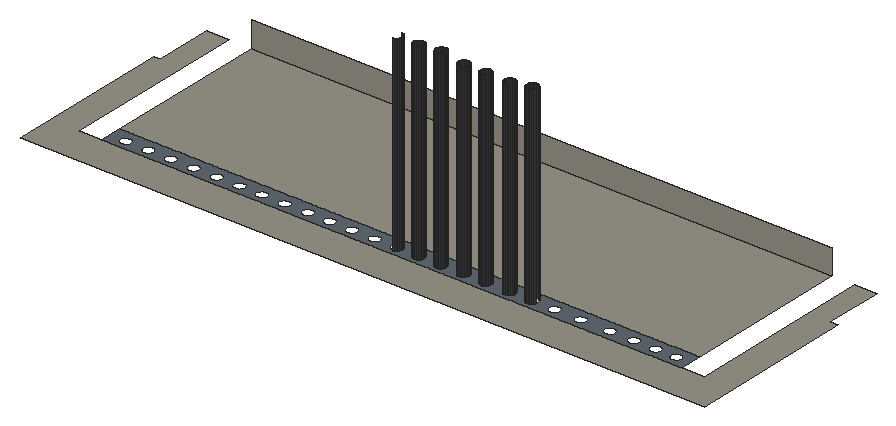
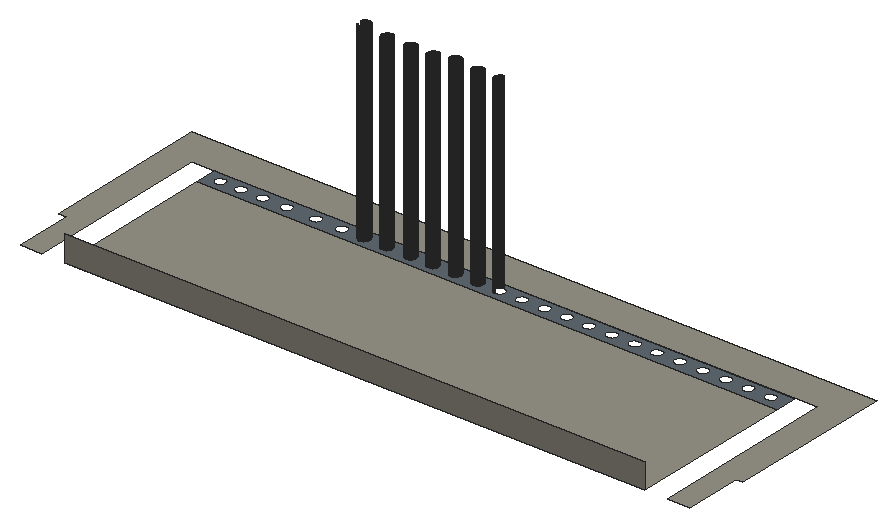
# SketchUp Ruby script. Lengths in inches.
U = 1.inch
M = Sketchup.active_model
def pt(a) = Geom::Point3d.new(a.map { |v| v * U })
def face(e, loops, mat)
  f = e.add_face(loops[0].map { |a| pt(a) })
  loops[1..].each { |l| e.add_face(l.map { |a| pt(a) }).erase! }
  f.material = f.back_material = mat if mat
  f
end
# faces: each face lists its corners as indices into pts; further lists are holes
def faces(e, pts, list, mat = nil) = list.each { |f| face(e, (f[0].is_a?(Array) ? f : [f]).map { |l| l.map { |i| pts[i] } }, mat) }
# xy, xz, yz: faces in a plane at the given z, y or x. An outline is a flat list of corners, or four numbers for a rectangle; further outlines are holes
def ring(l) = l.size == 4 ? [[l[0], l[1]], [l[2], l[1]], [l[2], l[3]], [l[0], l[3]]] : l.each_slice(2).to_a
def flat(e, list, mat, &to3) = list.each { |f| face(e, (f[0].is_a?(Array) ? f : [f]).map { |l| ring(l).map { |u, v| to3.(u, v) } }, mat) }
def xy(e, z, list, mat = nil) = flat(e, list, mat) { |x, y| [x, y, z] }
def xz(e, y, list, mat = nil) = flat(e, list, mat) { |x, z| [x, y, z] }
def yz(e, x, list, mat = nil) = flat(e, list, mat) { |y, z| [x, y, z] }
def lines(e, pts, list) = list.each { |a, b| e.add_line(pt(pts[a]), pt(pts[b])) }
# prism: a flat outline (further loops are holes) pulled along v
def prism(e, loops, v, mat = nil)
  f = face(e, loops, mat); d = Geom::Vector3d.new(v.map { |x| x * U })
  f.pushpull(f.normal.samedirection?(d) ? d.length : -d.length)
end
def box(e, o, s, mat = nil) = prism(e, [[o, [o[0] + s[0], o[1], o[2]], [o[0] + s[0], o[1] + s[1], o[2]], [o[0], o[1] + s[1], o[2]]]], [0, 0, s[2]], mat)
def at(x, y, z, deg = 0) = Geom::Transformation.translation(pt([x, y, z])) * Geom::Transformation.rotation(ORIGIN, Z_AXIS, deg.degrees)
def axes(o, x, y, z) = Geom::Transformation.new([*x, 0, *y, 0, *z, 0, *pt(o).to_a, 1])
def part(name) = M.definitions.add(name)
# library, detail: a bought-in or finely detailed component or shape, given as its bounding box
def library(name, o, s) = part(name).tap { |d| box(d.entities, o, s) }
def detail(e, o, s) = box(e.add_group.entities, o, s)
def put(e, d, t, mat = nil) = e.add_instance(d, t).tap { |i| i.material = mat if mat }
def group(e, t, mat = nil) = e.add_group.tap { |g| g.transformation = t; g.material = mat if mat }.entities
root = M.entities
M.materials.add("[Color M07]").color = [58, 58, 58]
M.materials.add("[Formica Graystone]").color = [149, 146, 135]
M.materials.add("[Formica Speckled Grey]").color = [94, 105, 111]
xy(root,334.79,[[262.29,121.51,262.12,121.56,261.96,121.65,261.84,121.78,261.75,121.93,261.71,122.11,261.71,122.28,261.76,122.46,261.85,122.61,261.98,122.74,262.13,122.83,262.31,122.87,262.48,122.87,262.66,122.82,262.8125,122.73,262.9375,122.6,263.03,122.45,263.07,122.27,263.07,122.09,263.02,121.92,262.93,121.76,262.8,121.64,262.65,121.55,262.47,121.51],[265.04,121.51,264.87,121.56,264.71,121.65,264.59,121.78,264.5,121.93,264.46,122.11,264.46,122.28,264.51,122.46,264.6,122.61,264.73,122.74,264.88,122.83,265.06,122.87,265.23,122.87,265.41,122.82,265.5625,122.73,265.6875,122.6,265.78,122.45,265.82,122.27,265.82,122.09,265.77,121.92,265.68,121.76,265.55,121.64,265.4,121.55,265.22,121.51],[267.79,121.51,267.62,121.56,267.46,121.65,267.34,121.78,267.25,121.93,267.21,122.11,267.21,122.28,267.26,122.46,267.35,122.61,267.48,122.74,267.63,122.83,267.81,122.87,267.98,122.87,268.16,122.82,268.3125,122.73,268.4375,122.6,268.53,122.45,268.57,122.27,268.57,122.09,268.52,121.92,268.43,121.76,268.3,121.64,268.15,121.55,267.97,121.51],[270.54,121.51,270.37,121.56,270.21,121.65,270.09,121.78,270,121.93,269.96,122.11,269.96,122.28,270.01,122.46,270.1,122.61,270.23,122.74,270.38,122.83,270.56,122.87,270.73,122.87,270.91,122.82,271.0625,122.73,271.1875,122.6,271.28,122.45,271.32,122.27,271.32,122.09,271.27,121.92,271.18,121.76,271.05,121.64,270.9,121.55,270.72,121.51],[273.48,121.51,273.31,121.56,273.15,121.65,273.03,121.78,272.9375,121.93,272.89,122.11,272.9,122.28,272.94,122.46,273.03,122.61,273.16,122.74,273.32,122.83,273.49,122.87,273.67,122.87,273.85,122.82,274,122.73,274.125,122.6,274.21,122.45,274.26,122.27,274.26,122.09,274.21,121.92,274.12,121.76,273.99,121.64,273.83,121.55,273.66,121.51],
  [276.29,121.51,276.12,121.56,275.96,121.65,275.84,121.78,275.75,121.93,275.71,122.11,275.71,122.28,275.76,122.46,275.85,122.61,275.98,122.74,276.13,122.83,276.31,122.87,276.48,122.87,276.66,122.82,276.8125,122.73,276.9375,122.6,277.03,122.45,277.07,122.27,277.07,122.09,277.02,121.92,276.93,121.76,276.8,121.64,276.65,121.55,276.47,121.51]])
xy(root,334.79,[[217.8,116.35,302.43,116.35,302.43,136.91,301.43,136.91,301.43,144.04,298.73,144.04,298.73,120.91,221.4,120.91,221.4,144.04,218.68,144.04,218.68,136.91,217.8,136.91],[224.22,123.73,295.92,144.04]],"[Formica Graystone]")
xy(root,334.79,[[[224.22,120.91,295.92,123.73],[228.85,121.51,228.68,121.56,228.53,121.65,228.4,121.78,228.3125,121.93,228.27,122.11,228.27,122.28,228.32,122.46,228.41,122.61,228.54,122.74,228.69,122.83,228.87,122.87,229.05,122.87,229.22,122.82,229.375,122.73,229.5,122.6,229.59,122.45,229.63,122.27,229.63,122.09,229.58,121.92,229.49,121.76,229.36,121.64,229.21,121.55,229.03,121.51],[231.67,121.51,231.49,121.56,231.34,121.65,231.21,121.78,231.125,121.93,231.08,122.11,231.08,122.28,231.13,122.46,231.22,122.61,231.35,122.74,231.51,122.83,231.68,122.87,231.86,122.87,232.03,122.82,232.1875,122.73,232.3125,122.6,232.4,122.45,232.45,122.27,232.44,122.09,232.4,121.92,232.3,121.76,232.18,121.64,232.02,121.55,231.85,121.51],[234.48,121.51,234.31,121.56,234.15,121.65,234.03,121.78,233.9375,121.93,233.89,122.11,233.9,122.28,233.94,122.46,234.03,122.61,234.16,122.74,234.32,122.83,234.49,122.87,234.67,122.87,234.85,122.82,235,122.73,235.125,122.6,235.21,122.45,235.26,122.27,235.26,122.09,235.21,121.92,235.12,121.76,234.99,121.64,234.83,121.55,234.66,121.51],[237.29,121.51,237.12,121.56,236.96,121.65,236.84,121.78,236.75,121.93,236.71,122.11,236.71,122.28,236.76,122.46,236.85,122.61,236.98,122.74,237.13,122.83,237.31,122.87,237.48,122.87,237.66,122.82,237.8125,122.73,237.9375,122.6,238.03,122.45,238.07,122.27,238.07,122.09,238.02,121.92,237.93,121.76,237.8,121.64,237.65,121.55,237.47,121.51],[240.1,121.51,239.93,121.56,239.78,121.65,239.65,121.78,239.5625,121.93,239.52,122.11,239.52,122.28,239.57,122.46,239.66,122.61,239.79,122.74,239.94,122.83,240.12,122.87,240.3,122.87,240.47,122.82,240.625,122.73,240.75,122.6,240.84,122.45,240.88,122.27,240.88,122.09,240.83,121.92,240.74,121.76,240.61,121.64,240.46,121.55,240.28,121.51],[242.92,121.51,242.74,121.56,242.59,121.65,242.46,121.78,242.375,121.93,242.33,122.11,242.33,122.28,242.38,122.46,242.47,122.61,242.6,122.74,242.76,122.83,242.93,122.87,243.11,122.87,243.28,122.82,243.4375,122.73,243.5625,122.6,243.65,122.45,243.7,122.27,243.69,122.09,243.65,121.92,243.55,121.76,243.43,121.64,243.27,121.55,243.1,121.51],[245.73,121.51,245.56,121.56,245.4,121.65,245.28,121.78,245.1875,121.93,245.14,122.11,245.15,122.28,245.19,122.46,245.28,122.61,245.41,122.74,245.57,122.83,245.74,122.87,245.92,122.87,246.1,122.82,246.25,122.73,246.375,122.6,246.46,122.45,246.51,122.27,246.51,122.09,246.46,121.92,246.37,121.76,246.24,121.64,246.08,121.55,245.91,121.51],[248.54,121.51,248.37,121.56,248.21,121.65,248.09,121.78,248,121.93,247.96,122.11,247.96,122.28,248.01,122.46,248.1,122.61,248.23,122.74,248.38,122.83,248.56,122.87,248.73,122.87,248.91,122.82,249.0625,122.73,249.1875,122.6,249.28,122.45,249.32,122.27,249.32,122.09,249.27,121.92,249.18,121.76,249.05,121.64,248.9,121.55,248.72,121.51],[251.29,121.51,251.12,121.56,250.96,121.65,250.84,121.78,250.75,121.93,250.71,122.11,250.71,122.28,250.76,122.46,250.85,122.61,250.98,122.74,251.13,122.83,251.31,122.87,251.48,122.87,251.66,122.82,251.8125,122.73,251.9375,122.6,252.03,122.45,252.07,122.27,252.07,122.09,252.02,121.92,251.93,121.76,251.8,121.64,251.65,121.55,251.47,121.51],[254.04,121.51,253.87,121.56,253.71,121.65,253.59,121.78,253.5,121.93,253.46,122.11,253.46,122.28,253.51,122.46,253.6,122.61,253.73,122.74,253.88,122.83,254.06,122.87,254.23,122.87,254.41,122.82,254.5625,122.73,254.6875,122.6,254.78,122.45,254.82,122.27,254.82,122.09,254.77,121.92,254.68,121.76,254.55,121.64,254.4,121.55,254.22,121.51],[256.79,121.51,256.62,121.56,256.46,121.65,256.34,121.78,256.25,121.93,256.21,122.11,256.21,122.28,256.26,122.46,256.35,122.61,256.48,122.74,256.63,122.83,256.81,122.87,256.98,122.87,257.16,122.82,257.3125,122.73,257.4375,122.6,257.53,122.45,257.57,122.27,257.57,122.09,257.52,121.92,257.43,121.76,257.3,121.64,257.15,121.55,256.97,121.51],[259.54,121.51,259.37,121.56,259.21,121.65,259.09,121.78,259,121.93,258.96,122.11,258.96,122.28,259.01,122.46,259.1,122.61,259.23,122.74,259.38,122.83,259.56,122.87,259.73,122.87,259.91,122.82,260.0625,122.73,260.1875,122.6,260.28,122.45,260.32,122.27,260.32,122.09,260.27,121.92,260.18,121.76,260.05,121.64,259.9,121.55,259.72,121.51],[262.29,121.51,262.12,121.56,261.96,121.65,261.84,121.78,261.75,121.93,261.71,122.11,261.71,122.28,261.76,122.46,261.85,122.61,261.98,122.74,262.13,122.83,262.31,122.87,262.48,122.87,262.66,122.82,262.8125,122.73,262.9375,122.6,263.03,122.45,263.07,122.27,263.07,122.09,263.02,121.92,262.93,121.76,262.8,121.64,262.65,121.55,262.47,121.51],[265.04,121.51,264.87,121.56,264.71,121.65,264.59,121.78,264.5,121.93,264.46,122.11,264.46,122.28,264.51,122.46,264.6,122.61,264.73,122.74,264.88,122.83,265.06,122.87,265.23,122.87,265.41,122.82,265.5625,122.73,265.6875,122.6,265.78,122.45,265.82,122.27,265.82,122.09,265.77,121.92,265.68,121.76,265.55,121.64,265.4,121.55,265.22,121.51],[267.79,121.51,267.62,121.56,267.46,121.65,267.34,121.78,267.25,121.93,267.21,122.11,267.21,122.28,267.26,122.46,267.35,122.61,267.48,122.74,267.63,122.83,267.81,122.87,267.98,122.87,268.16,122.82,268.3125,122.73,268.4375,122.6,268.53,122.45,268.57,122.27,268.57,122.09,268.52,121.92,268.43,121.76,268.3,121.64,268.15,121.55,267.97,121.51],[270.54,121.51,270.37,121.56,270.21,121.65,270.09,121.78,270,121.93,269.96,122.11,269.96,122.28,270.01,122.46,270.1,122.61,270.23,122.74,270.38,122.83,270.56,122.87,270.73,122.87,270.91,122.82,271.0625,122.73,271.1875,122.6,271.28,122.45,271.32,122.27,271.32,122.09,271.27,121.92,271.18,121.76,271.05,121.64,270.9,121.55,270.72,121.51],[294.1,121.51,293.93,121.56,293.78,121.65,293.65,121.78,293.5625,121.93,293.52,122.11,293.52,122.28,293.57,122.46,293.66,122.61,293.79,122.74,293.94,122.83,294.12,122.87,294.3,122.87,294.47,122.82,294.625,122.73,294.75,122.6,294.84,122.45,294.88,122.27,294.88,122.09,294.83,121.92,294.74,121.76,294.61,121.64,294.46,121.55,294.28,121.51],[273.48,121.51,273.31,121.56,273.15,121.65,273.03,121.78,272.9375,121.93,272.89,122.11,272.9,122.28,272.94,122.46,273.03,122.61,273.16,122.74,273.32,122.83,273.49,122.87,273.67,122.87,273.85,122.82,274,122.73,274.125,122.6,274.21,122.45,274.26,122.27,274.26,122.09,274.21,121.92,274.12,121.76,273.99,121.64,273.83,121.55,273.66,121.51],[291.54,121.51,291.37,121.56,291.21,121.65,291.09,121.78,291,121.93,290.96,122.11,290.96,122.28,291.01,122.46,291.1,122.61,291.23,122.74,291.38,122.83,291.56,122.87,291.73,122.87,291.91,122.82,292.0625,122.73,292.1875,122.6,292.28,122.45,292.32,122.27,292.32,122.09,292.27,121.92,292.18,121.76,292.05,121.64,291.9,121.55,291.72,121.51],[276.29,121.51,276.12,121.56,275.96,121.65,275.84,121.78,275.75,121.93,275.71,122.11,275.71,122.28,275.76,122.46,275.85,122.61,275.98,122.74,276.13,122.83,276.31,122.87,276.48,122.87,276.66,122.82,276.8125,122.73,276.9375,122.6,277.03,122.45,277.07,122.27,277.07,122.09,277.02,121.92,276.93,121.76,276.8,121.64,276.65,121.55,276.47,121.51],[288.85,121.51,288.68,121.56,288.53,121.65,288.4,121.78,288.3125,121.93,288.27,122.11,288.27,122.28,288.32,122.46,288.41,122.61,288.54,122.74,288.69,122.83,288.87,122.87,289.05,122.87,289.22,122.82,289.375,122.73,289.5,122.6,289.59,122.45,289.63,122.27,289.63,122.09,289.58,121.92,289.49,121.76,289.36,121.64,289.21,121.55,289.03,121.51],[279.04,121.51,278.87,121.56,278.71,121.65,278.59,121.78,278.5,121.93,278.46,122.11,278.46,122.28,278.51,122.46,278.6,122.61,278.73,122.74,278.88,122.83,279.06,122.87,279.23,122.87,279.41,122.82,279.5625,122.73,279.6875,122.6,279.78,122.45,279.82,122.27,279.82,122.09,279.77,121.92,279.68,121.76,279.55,121.64,279.4,121.55,279.22,121.51],[285.92,121.51,285.74,121.56,285.59,121.65,285.46,121.78,285.375,121.93,285.33,122.11,285.33,122.28,285.38,122.46,285.47,122.61,285.6,122.74,285.76,122.83,285.93,122.87,286.11,122.87,286.28,122.82,286.4375,122.73,286.5625,122.6,286.65,122.45,286.7,122.27,286.69,122.09,286.65,121.92,286.55,121.76,286.43,121.64,286.27,121.55,286.1,121.51],[282.29,121.51,282.12,121.56,281.96,121.65,281.84,121.78,281.75,121.93,281.71,122.11,281.71,122.28,281.76,122.46,281.85,122.61,281.98,122.74,282.13,122.83,282.31,122.87,282.48,122.87,282.66,122.82,282.8125,122.73,282.9375,122.6,283.03,122.45,283.07,122.27,283.07,122.09,283.02,121.92,282.93,121.76,282.8,121.64,282.65,121.55,282.47,121.51],[226.04,121.51,225.87,121.56,225.71,121.65,225.59,121.78,225.5,121.93,225.46,122.11,225.46,122.28,225.51,122.46,225.6,122.61,225.73,122.74,225.88,122.83,226.06,122.87,226.23,122.87,226.41,122.82,226.5625,122.73,226.6875,122.6,226.78,122.45,226.82,122.27,226.82,122.09,226.77,121.92,226.68,121.76,226.55,121.64,226.4,121.55,226.22,121.51]]],"[Formica Speckled Grey]")
xz(root,121.51,[[262.29,334.79,262.47,358.31],[265.04,334.79,265.22,358.53],[267.79,334.79,267.97,358.07],[270.54,334.79,270.72,358.07],[273.48,334.79,273.66,358.07],
  [276.29,334.79,276.47,358.53]],"[Color M07]")
xz(root,122.87,[[262.31,334.79,262.48,358.31],[265.06,334.79,265.23,358.53],[267.81,334.79,267.98,358.07],[270.56,334.79,270.73,358.07],[273.49,334.79,273.67,358.07],
  [276.31,334.79,276.48,358.53]],"[Color M07]")
xz(root,144.04,[[224.22,334.79,295.92,337.93]],"[Formica Graystone]")
yz(root,260.32,[[122.09,334.79,122.27,358.31]],"[Color M07]")
yz(root,261.71,[[122.11,334.79,122.28,358.31]],"[Color M07]")
yz(root,263.07,[[122.09,334.79,122.27,358.31]],"[Color M07]")
yz(root,264.46,[[122.11,334.79,122.28,358.53]],"[Color M07]")
yz(root,265.82,[[122.09,334.79,122.27,358.53]],"[Color M07]")
yz(root,267.21,[[122.11,334.79,122.28,358.07]],"[Color M07]")
yz(root,268.57,[[122.09,334.79,122.27,358.07]],"[Color M07]")
yz(root,269.96,[[122.11,334.79,122.28,358.07]],"[Color M07]")
yz(root,271.32,[[122.09,334.79,122.27,358.07]],"[Color M07]")
yz(root,274.26,[[122.09,334.79,122.27,358.07]],"[Color M07]")
yz(root,275.71,[[122.11,334.79,122.28,358.53]],"[Color M07]")
p = [[259.72,121.51,334.79],[259.9,121.55,334.79],[259.9,121.55,358.31],[259.72,121.51,358.31],[262.12,121.56,334.79],[262.29,121.51,334.79],
  [262.29,121.51,358.31],[262.12,121.56,358.31],[262.12,121.56,357.4],[262.47,121.51,334.79],[262.65,121.55,334.79],[262.65,121.55,358.31],
  [262.47,121.51,358.31],[264.87,121.56,334.79],[265.04,121.51,334.79],[265.04,121.51,358.53],[264.87,121.56,358.53],[264.87,121.56,357.4],
  [265.22,121.51,334.79],[265.4,121.55,334.79],[265.4,121.55,358.53],[265.22,121.51,358.53],[267.62,121.56,334.79],[267.79,121.51,334.79],
  [267.79,121.51,358.07],[267.62,121.56,358.07],[267.62,121.56,357.4],[267.97,121.51,334.79],[268.15,121.55,334.79],[268.15,121.55,358.07],
  [267.97,121.51,358.07],[270.37,121.56,334.79],[270.54,121.51,334.79],[270.54,121.51,358.07],[270.37,121.56,358.07],[270.37,121.56,357.4],
  [270.72,121.51,334.79],[270.9,121.55,334.79],[270.9,121.55,358.07],[270.72,121.51,358.07],[273.31,121.56,334.79],[273.48,121.51,334.79],
  [273.48,121.51,358.07],[273.31,121.56,358.07],[273.31,121.56,357.4],[273.66,121.51,334.79],[273.83,121.55,334.79],[273.83,121.55,358.07],
  [273.66,121.51,358.07],[276.12,121.56,334.79],[276.29,121.51,334.79],[276.29,121.51,358.53],[276.12,121.56,358.53],[276.12,121.56,357.4],
  [276.47,121.51,334.79],[276.65,121.55,334.79],[276.65,121.55,358.53],[276.47,121.51,358.53],[260.05,121.64,334.79],[260.05,121.64,358.31],
  [260.18,121.76,334.79],[260.18,121.76,358.31],[261.84,121.78,334.79],[261.96,121.65,334.79],[261.96,121.65,358.31],[261.84,121.78,358.31],
  [262.8,121.64,334.79],[262.8,121.64,358.31],[262.93,121.76,334.79],[262.93,121.76,358.31],[264.59,121.78,334.79],[264.71,121.65,334.79],
  [264.71,121.65,358.53],[264.59,121.78,358.53],[265.55,121.64,334.79],[265.55,121.64,358.53],[265.68,121.76,334.79],[265.68,121.76,358.53],
  [267.34,121.78,334.79],[267.46,121.65,334.79],[267.46,121.65,358.07],[267.34,121.78,358.07],[268.3,121.64,334.79],[268.3,121.64,358.07],
  [268.43,121.76,334.79],[268.43,121.76,358.07],[270.09,121.78,334.79],[270.21,121.65,334.79],[270.21,121.65,358.07],[270.09,121.78,358.07],
  [271.05,121.64,334.79],[271.05,121.64,358.07],[271.18,121.76,334.79],[271.18,121.76,358.07],[273.03,121.78,334.79],[273.15,121.65,334.79],
  [273.15,121.65,358.07],[273.03,121.78,358.07],[273.99,121.64,334.79],[273.99,121.64,358.07],[274.12,121.76,334.79],[274.12,121.76,358.07],
  [275.84,121.78,334.79],[275.96,121.65,334.79],[275.96,121.65,358.53],[275.84,121.78,358.53],[276.8,121.64,334.79],[276.8,121.64,358.53],
  [276.93,121.76,334.79],[276.93,121.76,358.53],[260.27,121.92,334.79],[260.27,121.92,358.31],[261.75,121.93,334.79],[261.75,121.93,358.31],
  [263.02,121.92,334.79],[263.02,121.92,358.31],[264.5,121.93,334.79],[264.5,121.93,358.53],[265.77,121.92,334.79],[265.77,121.92,358.53],
  [267.25,121.93,334.79],[267.25,121.93,358.07],[268.52,121.92,334.79],[268.52,121.92,358.07],[270,121.93,334.79],[270,121.93,358.07],
  [271.27,121.92,334.79],[271.27,121.92,358.07],[272.9375,121.93,334.79],[272.9375,121.93,358.07],[274.21,121.92,334.79],[274.21,121.92,358.07],
  [275.75,121.93,334.79],[275.75,121.93,358.53],[277.02,121.92,334.79],[277.02,121.92,358.53],[260.32,122.09,334.79],[260.32,122.09,358.31],
  [261.71,122.11,334.79],[261.71,122.11,358.31],[263.07,122.09,334.79],[263.07,122.09,358.31],[264.46,122.11,334.79],[264.46,122.11,358.53],
  [265.82,122.09,334.79],[265.82,122.09,358.53],[267.21,122.11,334.79],[267.21,122.11,358.07],[268.57,122.09,334.79],[268.57,122.09,358.07],
  [269.96,122.11,334.79],[269.96,122.11,358.07],[271.32,122.09,334.79],[271.32,122.09,358.07],[272.89,122.11,334.79],[272.89,122.11,358.07],
  [274.26,122.09,334.79],[274.26,122.09,358.07],[275.71,122.11,334.79],[275.71,122.11,358.53],[272.9,122.28,334.79],[272.9,122.28,358.07],
  [260.32,122.27,334.79],[260.28,122.45,334.79],[260.28,122.45,358.31],[260.32,122.27,358.31],[261.76,122.46,334.79],[261.71,122.28,334.79],
  [261.71,122.28,358.31],[261.76,122.46,358.31],[263.07,122.27,334.79],[263.03,122.45,334.79],[263.03,122.45,358.31],[263.07,122.27,358.31],
  [264.51,122.46,334.79],[264.46,122.28,334.79],[264.46,122.28,358.53],[264.51,122.46,358.53],[265.82,122.27,334.79],[265.78,122.45,334.79],
  [265.78,122.45,358.53],[265.82,122.27,358.53],[267.26,122.46,334.79],[267.21,122.28,334.79],[267.21,122.28,358.07],[267.26,122.46,358.07],
  [268.57,122.27,334.79],[268.53,122.45,334.79],[268.53,122.45,358.07],[268.57,122.27,358.07],[270.01,122.46,334.79],[269.96,122.28,334.79],
  [269.96,122.28,358.07],[270.01,122.46,358.07],[271.32,122.27,334.79],[271.28,122.45,334.79],[271.28,122.45,358.07],[271.32,122.27,358.07],
  [272.94,122.46,334.79],[272.94,122.46,358.07],[274.26,122.27,334.79],[274.21,122.45,334.79],[274.21,122.45,358.07],[274.26,122.27,358.07],
  [275.76,122.46,334.79],[275.71,122.28,334.79],[275.71,122.28,358.53],[275.76,122.46,358.53],[260.1875,122.6,334.79],[260.1875,122.6,358.31],
  [262.9375,122.6,334.79],[262.9375,122.6,358.31],[265.6875,122.6,334.79],[265.6875,122.6,358.53],[268.4375,122.6,334.79],[268.4375,122.6,358.07],
  [271.1875,122.6,334.79],[271.1875,122.6,358.07],[274.125,122.6,334.79],[274.125,122.6,358.07],[261.85,122.61,334.79],[261.85,122.61,358.31],
  [264.6,122.61,334.79],[264.6,122.61,358.53],[267.35,122.61,334.79],[267.35,122.61,358.07],[270.1,122.61,334.79],[270.1,122.61,358.07],
  [273.03,122.61,334.79],[273.03,122.61,358.07],[275.85,122.61,334.79],[275.85,122.61,358.53],[260.0625,122.73,334.79],[260.0625,122.73,358.31],
  [261.98,122.74,334.79],[261.98,122.74,358.31],[262.8125,122.73,334.79],[262.8125,122.73,358.31],[264.73,122.74,334.79],[264.73,122.74,358.53],
  [265.5625,122.73,334.79],[265.5625,122.73,358.53],[267.48,122.74,334.79],[267.48,122.74,358.07],[268.3125,122.73,334.79],[268.3125,122.73,358.07],
  [270.23,122.74,334.79],[270.23,122.74,358.07],[271.0625,122.73,334.79],[271.0625,122.73,358.07],[273.16,122.74,334.79],[273.16,122.74,358.07],
  [274,122.73,334.79],[274,122.73,358.07],[275.98,122.74,334.79],[275.98,122.74,358.53],[276.9375,122.6,334.79],[276.8125,122.73,334.79],
  [276.8125,122.73,358.53],[276.9375,122.6,358.53],[259.91,122.82,334.79],[259.91,122.82,358.31],[262.13,122.83,334.79],[262.13,122.83,358.31],
  [262.66,122.82,334.79],[262.66,122.82,358.31],[264.88,122.83,334.79],[264.88,122.83,358.53],[265.41,122.82,334.79],[265.41,122.82,358.53],
  [267.63,122.83,334.79],[267.63,122.83,358.07],[268.16,122.82,334.79],[268.16,122.82,358.07],[270.38,122.83,334.79],[270.38,122.83,358.07],
  [270.91,122.82,334.79],[270.91,122.82,358.07],[273.32,122.83,334.79],[273.32,122.83,358.07],[273.85,122.82,334.79],[273.85,122.82,358.07],
  [276.13,122.83,334.79],[276.13,122.83,358.53],[276.66,122.82,334.79],[276.66,122.82,358.53],[259.73,122.87,334.79],[259.73,122.87,358.31],
  [262.31,122.87,334.79],[262.31,122.87,358.31],[262.48,122.87,334.79],[262.48,122.87,358.31],[265.06,122.87,334.79],[265.06,122.87,358.53],
  [265.23,122.87,334.79],[265.23,122.87,358.53],[267.81,122.87,334.79],[267.81,122.87,358.07],[267.98,122.87,334.79],[267.98,122.87,358.07],
  [270.56,122.87,334.79],[270.56,122.87,358.07],[270.73,122.87,334.79],[270.73,122.87,358.07],[273.49,122.87,334.79],[273.49,122.87,358.07],
  [273.67,122.87,334.79],[273.67,122.87,358.07],[276.31,122.87,334.79],[276.31,122.87,358.53],[276.48,122.87,334.79],[276.48,122.87,358.53]]
faces(root,p,[[0,1,2,3],[4,5,6,7,8],[9,10,11,12],[13,14,15,16,17],[18,19,20,21],[22,23,24,25,26],[27,28,29,30],[31,32,33,34,35],
  [36,37,38,39],[40,41,42,43,44],[45,46,47,48],[49,50,51,52,53],[54,55,56,57],[1,58,59,2],[58,60,61,59],[62,63,64,65],
  [63,4,8,7,64],[10,66,67,11],[66,68,69,67],[70,71,72,73],[71,13,17,16,72],[19,74,75,20],[74,76,77,75],[78,79,80,81],
  [79,22,26,25,80],[28,82,83,29],[82,84,85,83],[86,87,88,89],[87,31,35,34,88],[37,90,91,38],[90,92,93,91],[94,95,96,97],
  [95,40,44,43,96],[46,98,99,47],[98,100,101,99],[102,103,104,105],[103,49,53,52,104],[55,106,107,56],[106,108,109,107],[60,110,111,61],
  [112,62,65,113],[68,114,115,69],[116,70,73,117],[76,118,119,77],[120,78,81,121],[84,122,123,85],[124,86,89,125],[92,126,127,93],
  [128,94,97,129],[100,130,131,101],[132,102,105,133],[108,134,135,109],[110,136,137,111],[138,112,113,139],[114,140,141,115],[142,116,117,143],
  [118,144,145,119],[146,120,121,147],[122,148,149,123],[150,124,125,151],[126,152,153,127],[154,128,129,155],[130,156,157,131],[158,132,133,159],
  [160,154,155,161],[162,163,164,165],[166,167,168,169],[170,171,172,173],[174,175,176,177],[178,179,180,181],[182,183,184,185],[186,187,188,189],
  [190,191,192,193],[194,195,196,197],[198,160,161,199],[200,201,202,203],[204,205,206,207],[163,208,209,164],[171,210,211,172],[179,212,213,180],
  [187,214,215,188],[195,216,217,196],[201,218,219,202],[220,166,169,221],[222,174,177,223],[224,182,185,225],[226,190,193,227],[228,198,199,229],
  [230,204,207,231],[208,232,233,209],[234,220,221,235],[210,236,237,211],[238,222,223,239],[212,240,241,213],[242,224,225,243],[214,244,245,215],
  [246,226,227,247],[216,248,249,217],[250,228,229,251],[218,252,253,219],[254,230,231,255],[256,257,258,259],[232,260,261,233],[262,234,235,263],
  [236,264,265,237],[266,238,239,267],[240,268,269,241],[270,242,243,271],[244,272,273,245],[274,246,247,275],[248,276,277,249],[278,250,251,279],
  [252,280,281,253],[282,254,255,283],[257,284,285,258],[260,286,287,261],[288,262,263,289],[264,290,291,265],[292,266,267,293],[268,294,295,269],
  [296,270,271,297],[272,298,299,273],[300,274,275,301],[276,302,303,277],[304,278,279,305],[280,306,307,281],[308,282,283,309],[284,310,311,285]],"[Color M07]")
